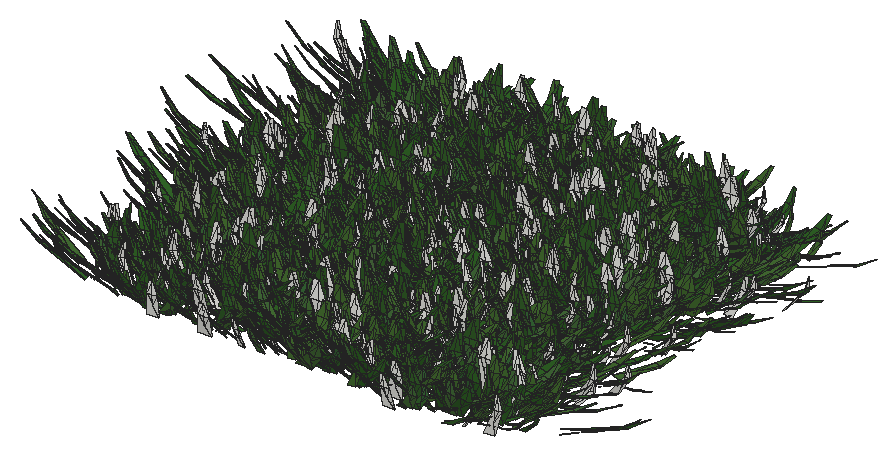
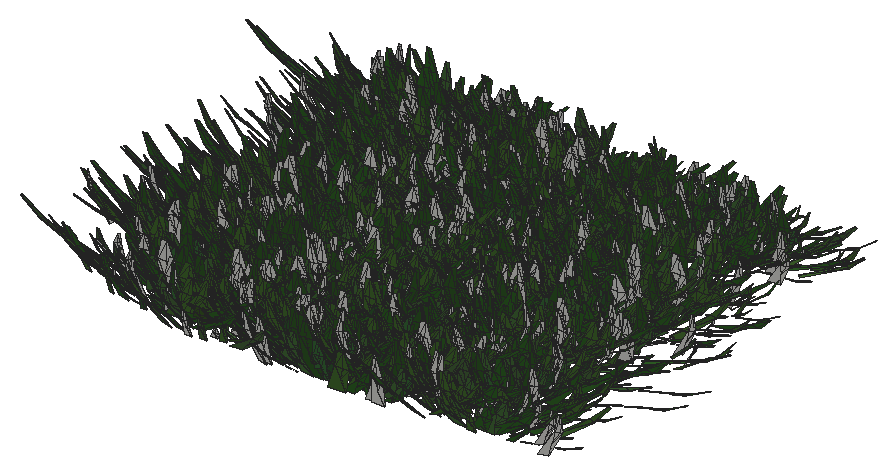
# SketchUp Ruby script. Lengths in inches.
U = 1.inch
M = Sketchup.active_model
def pt(a) = Geom::Point3d.new(a.map { |v| v * U })
def face(e, loops, mat)
  f = e.add_face(loops[0].map { |a| pt(a) })
  loops[1..].each { |l| e.add_face(l.map { |a| pt(a) }).erase! }
  f.material = f.back_material = mat if mat
  f
end
# faces: each face lists its corners as indices into pts; further lists are holes
def faces(e, pts, list, mat = nil) = list.each { |f| face(e, (f[0].is_a?(Array) ? f : [f]).map { |l| l.map { |i| pts[i] } }, mat) }
# xy, xz, yz: faces in a plane at the given z, y or x. An outline is a flat list of corners, or four numbers for a rectangle; further outlines are holes
def ring(l) = l.size == 4 ? [[l[0], l[1]], [l[2], l[1]], [l[2], l[3]], [l[0], l[3]]] : l.each_slice(2).to_a
def flat(e, list, mat, &to3) = list.each { |f| face(e, (f[0].is_a?(Array) ? f : [f]).map { |l| ring(l).map { |u, v| to3.(u, v) } }, mat) }
def xy(e, z, list, mat = nil) = flat(e, list, mat) { |x, y| [x, y, z] }
def xz(e, y, list, mat = nil) = flat(e, list, mat) { |x, z| [x, y, z] }
def yz(e, x, list, mat = nil) = flat(e, list, mat) { |y, z| [x, y, z] }
def lines(e, pts, list) = list.each { |a, b| e.add_line(pt(pts[a]), pt(pts[b])) }
# prism: a flat outline (further loops are holes) pulled along v
def prism(e, loops, v, mat = nil)
  f = face(e, loops, mat); d = Geom::Vector3d.new(v.map { |x| x * U })
  f.pushpull(f.normal.samedirection?(d) ? d.length : -d.length)
end
def box(e, o, s, mat = nil) = prism(e, [[o, [o[0] + s[0], o[1], o[2]], [o[0] + s[0], o[1] + s[1], o[2]], [o[0], o[1] + s[1], o[2]]]], [0, 0, s[2]], mat)
def at(x, y, z, deg = 0) = Geom::Transformation.translation(pt([x, y, z])) * Geom::Transformation.rotation(ORIGIN, Z_AXIS, deg.degrees)
def axes(o, x, y, z) = Geom::Transformation.new([*x, 0, *y, 0, *z, 0, *pt(o).to_a, 1])
def part(name) = M.definitions.add(name)
# library, detail: a bought-in or finely detailed component or shape, given as its bounding box
def library(name, o, s) = part(name).tap { |d| box(d.entities, o, s) }
def detail(e, o, s) = box(e.add_group.entities, o, s)
def put(e, d, t, mat = nil) = e.add_instance(d, t).tap { |i| i.material = mat if mat }
def group(e, t, mat = nil) = e.add_group.tap { |g| g.transformation = t; g.material = mat if mat }.entities
root = M.entities
M.materials.add("Material10").color = [48, 100, 38]
M.materials.add("Material3").color = [68, 110, 58]
M.materials.add("Material4").color = [48, 90, 38]
M.materials.add("Material5").color = [68, 110, 48]
M.materials.add("Material6").color = [48, 90, 48]
M.materials.add("Material7").color = [58, 110, 58]
M.materials.add("Material8").color = [58, 90, 38]
M.materials.add("Material9").color = [68, 100, 58]
c1 = part("grass00")
p = [[-0.6875,0.15,0],[-0.56,0.08,5.52],[-0.04,0.03,2.76],[0.48,-0.02,0],[0.35,-0.02,5.52],[-0.1,-0.14,5.52],
  [-0.12,0.65,8.37],[-0.42,0.65,8.37]]
faces(c1.entities,p,[[0,1,2,3],[3,2,4],[1,5,2],[5,4,2],[1,6,5],[4,5,6],[7,6,1]])
c2 = part("Group16\#1")
put(c2.entities,c1,axes([1.44,-0.61,-0.01],[0.05352,0.12609,0],[-0.10704,0.04543,0.07239],[0.06664,-0.02828,0.11628]),"Material6")
put(c2.entities,c1,axes([0.76,-0.15,-0.01],[0.04676,0.24062,0],[-0.23162,0.04501,0.06642],[0.0652,-0.01267,0.23595]),"Material3")
put(c2.entities,c1,axes([0.79,0.01,-0.01],[-0.00606,0.34651,0],[-0.34381,-0.00602,0.0432],[0.04319,0.00076,0.34386]))
put(c2.entities,c1,axes([1,0.23,-0.01],[-0.07192,0.31144,0],[-0.28722,-0.06632,0.1236],[0.12043,0.02781,0.29478]),"Material5")
put(c2.entities,c1,axes([1.66,0.77,-0.01],[-0.13828,0.29651,0],[-0.21551,-0.1005,0.22471],[0.20365,0.09498,0.23779]),"Material10")
put(c2.entities,c1,axes([0.6875,0.52,-0.01],[-0.18126,0.24051,0],[-0.22746,-0.17142,0.09788],[0.07817,0.05891,0.28481]),"Material5")
put(c2.entities,c1,axes([0.68,0.78,-0.01],[-0.215,0.18688,0],[-0.12385,-0.14248,0.21334],[0.13995,0.16101,0.18878]),"Material3")
put(c2.entities,c1,axes([0.56,1,-0.01],[-0.13756,0.07624,0],[-0.06159,-0.11112,0.0927],[0.04494,0.08108,0.12705]),"Material5")
put(c2.entities,c1,axes([0.2,0.64,-0.01],[-0.23729,0.07254,0],[-0.05711,-0.18681,0.153],[0.04473,0.14632,0.19535]),"Material10")
put(c2.entities,c1,axes([0.0625,0.72,-0.01],[-0.28874,0.02525,0],[-0.02179,-0.24916,0.14647],[0.01276,0.14591,0.25012]),"Material3")
put(c2.entities,c1,axes([-0.08,0.62,-0.01],[-0.34089,-0.04187,0],[0.03255,-0.26504,0.216],[-0.02633,0.21439,0.26703]),"Material10")
put(c2.entities,c1,axes([-0.34,0.98,-0.01],[-0.14314,-0.0493,0],[0.04397,-0.12769,0.06843],[-0.02228,0.0647,0.13505]),"Material10")
put(c2.entities,c1,axes([-0.87,1.45,-0.01],[-0.23488,-0.14114,0],[0.13761,-0.22901,0.06087],[-0.03135,0.05217,0.26717]))
put(c2.entities,c1,axes([-0.72,0.77,-0.01],[-0.14208,-0.13251,0],[0.07209,-0.0773,0.16301],[-0.11118,0.11922,0.1057]),"Material10")
put(c2.entities,c1,axes([-0.62,0.43,-0.01],[-0.14845,-0.21203,0],[0.18654,-0.13061,0.12304],[-0.10079,0.07057,0.22772]),"Material3")
put(c2.entities,c1,axes([-0.68,0.29,-0.01],[-0.13639,-0.32136,0],[0.31723,-0.13464,0.05579],[-0.05136,0.0218,0.34462]),"Material4")
put(c2.entities,c1,axes([-0.64,0.125,-0.01],[-0.0458,-0.23569,0],[0.22124,-0.043,0.08276],[-0.08124,0.01579,0.22538]),"Material7")
put(c2.entities,c1,axes([-1.6,-0.03,-0.01],[0.00576,-0.32897,0],[0.27526,0.00482,0.18018],[-0.18015,-0.00315,0.2753]),"Material5")
put(c2.entities,c1,axes([-1.36,-0.31,-0.01],[0.05718,-0.24765,0],[0.18172,0.04196,0.17267],[-0.16825,-0.03885,0.1865]),"Material10")
put(c2.entities,c1,axes([-1.54,-0.72,-0.01],[0.06537,-0.14017,0],[0.13555,0.06321,0.03939],[-0.0357,-0.01665,0.14956]))
put(c2.entities,c1,axes([-1.19,-0.9,-0.01],[0.09597,-0.12735,0],[0.11214,0.08451,0.07557],[-0.06035,-0.04548,0.14042]),"Material9")
put(c2.entities,c1,axes([-0.47,-0.54,-0.01],[0.11588,-0.10072,0],[0.0618,0.0711,0.12124],[-0.07953,-0.0915,0.0942]))
put(c2.entities,c1,axes([-0.47,-0.84,-0.01],[0.11927,-0.0661,0],[0.06603,0.11913,0.00646],[-0.00313,-0.00565,0.13621]),"Material5")
put(c2.entities,c1,axes([-0.38,-1.24,-0.01],[0.28037,-0.08571,0],[0.0618,0.20215,0.20315],[-0.05939,-0.19428,0.21139]),"Material9")
put(c2.entities,c1,axes([-0.06,-0.66,-0.01],[0.22719,-0.01987,0],[0.01247,0.14255,0.17758],[-0.01547,-0.17691,0.1431]),"Material8")
put(c2.entities,c1,axes([0.11,-0.89,-0.01],[0.14882,0.01828,0],[-0.01058,0.08611,0.12229],[0.01491,-0.12138,0.08676]),"Material6")
put(c2.entities,c1,axes([0.25,-0.72,-0.01],[0.20481,0.07053,0],[-0.06206,0.18022,0.10291],[0.03351,-0.0973,0.1906]),"Material6")
put(c2.entities,c1,axes([0.85,-1.42,-0.01],[0.16481,0.09904,0],[-0.09472,0.15762,0.05616],[0.02893,-0.04814,0.18389]),"Material5")
put(c2.entities,c1,axes([1.01,-1.09,-0.01],[0.21858,0.20385,0],[-0.17495,0.1876,0.15339],[0.10462,-0.11218,0.25652]),"Material10")
put(c2.entities,c1,axes([1.01,-0.71,-0.01],[0.08733,0.12473,0],[-0.06445,0.04512,0.13037],[0.1068,-0.07477,0.07867]),"Material6")
c3 = part("Group15\#1")
put(c3.entities,c2,at(0,0,0))
c4 = part("3darcstudiotree_grass00\#1")
put(c4.entities,c3,at(0,0,0))
put(root,c4,axes([1026.98,934.91,0],[3.5158,-0.29291,0],[1.43894,1.07947,-0.01535],[0.02658,0.01994,1.5577]))
put(root,c4,axes([1028.4,963.98,0],[-3.60429,-0.54918,0],[1.97169,-0.80877,-0.03312],[0.12446,-0.05105,1.70984]))
put(root,c4,axes([1028.05,966.49,0],[1.08767,-1.10089,0],[4.34215,0.26813,-0.04714],[0.21998,0.01358,1.34372]))
put(root,c4,axes([1028.66,944.45,0],[-2.39381,-0.81809,0],[3.41436,-0.62442,-0.02018],[0.11154,-0.0204,1.81061]))
put(root,c4,axes([1027.22,954.21,0],[4.48845,-0.0996,0],[0.40703,1.14637,-0.01913],[0.01094,0.03082,1.86132]))
put(root,c4,axes([1029.08,960.92,0],[-2.33649,-0.74426,0],[3.77896,-0.74146,-0.04646],[0.22132,-0.04342,1.81816]))
put(root,c4,axes([1027.08,970.72,0],[3.85435,0.70628,0],[-2.80826,0.95783,-0.04132],[-0.15487,0.05282,1.88254]))
put(root,c4,axes([1027.89,945.71,0],[-1.94964,1.12405,0],[-4.22902,-0.45845,-0.00354],[-0.01854,-0.00201,1.64409]))
put(root,c4,axes([1027.61,969.89,0],[3.1818,0.67229,0],[-2.74348,0.81152,-0.00305],[-0.01175,0.00348,1.58836]))
put(root,c4,axes([1029.71,961.93,0],[-4.23791,0.69969,0],[-2.41225,-0.91316,-0.01955],[-0.05785,-0.0219,1.46911]))
put(root,c4,axes([1028.93,936.8,0],[3.32161,0.35112,0],[-1.50903,0.89222,-0.04149],[-0.12715,0.07518,1.90578]))
put(root,c4,axes([1028.85,937.58,0],[4.42522,0.39878,0],[-1.59159,1.10387,-0.05978],[-0.10331,0.07165,1.49495]))
put(root,c4,axes([1030.24,933.59,0],[-3.44676,0.28749,0],[-1.23509,-0.92549,-0.01591],[-0.0303,-0.02271,1.46774]))
put(root,c4,axes([1028.71,952.04,0],[3.38445,0.8074,0],[-3.01391,0.7896,-0.00767],[-0.03555,0.00931,1.8325]))
put(root,c4,axes([1029.99,939.57,0],[1.69893,-0.90725,0],[3.27841,0.3837,-0.04141],[0.32735,0.03831,1.97468]))
put(root,c4,axes([1029.22,965.58,0],[3.91819,0.15531,0],[-0.72225,1.13884,-0.02805],[-0.0304,0.04793,1.99488]))
put(root,c4,axes([1030.66,959.5625,0],[-4.474,0.54268,0],[-2.22283,-1.14534,-0.06144],[-0.11475,-0.05913,1.3618]))
put(root,c4,axes([1029.82,948.84,0],[4.53734,-0.32224,0],[1.09679,0.96521,-0.02465],[0.03792,0.03337,1.41248]))
put(root,c4,axes([1031.3,956,0],[-4.98405,0.08955,0],[-0.32681,-1.13684,-0.01837],[-0.00709,-0.02466,1.53349]))
put(root,c4,axes([1030.13,958.07,0],[-2.12527,0.78662,0],[-4.24604,-0.71699,-0.01862],[-0.09082,-0.01534,1.88514]))
put(root,c4,axes([1030.4,947.54,0],[-0.84491,0.92662,0],[-3.59657,-0.20496,-0.03421],[-0.27144,-0.01547,1.87625]))
put(root,c4,axes([1030.09,968.57,0],[4.27273,0.49757,0],[-1.69118,0.90766,-0.0112],[-0.0297,0.01594,1.5714]))
put(root,c4,axes([1030.77,950,0],[-2.09567,1.0755,0],[-4.66144,-0.56769,-0.00711],[-0.02652,-0.00323,1.34501]))
put(root,c4,axes([1031.4375,953.21,0],[3.76579,0.18942,0],[-0.73722,0.91603,-0.0192],[-0.02664,0.0331,1.64321]))
put(root,c4,axes([1033.09,937.56,0],[-4.50451,-0.0411,0],[0.16437,-1.12587,-0.04384],[0.00948,-0.0649,1.66887]))
put(root,c4,axes([1033.57,957.37,0],[1.13978,-1.18562,0],[3.93385,0.23636,-0.00397],[0.02802,0.00168,1.83602]))
put(root,c4,axes([1033.1875,968.22,0],[2.04927,-1.15149,0],[3.67293,0.40854,-0.03607],[0.18559,0.02064,1.41495]))
put(root,c4,axes([1033.99,936.09,0],[-3.89235,0.6193,0],[-1.97046,-0.77403,-0.04609],[-0.18429,-0.07239,1.7083]))
put(root,c4,axes([1034.17,961.06,0],[-4.69047,0.29817,0],[-0.94339,-0.92751,-0.01716],[-0.03313,-0.03258,1.87475]))
put(root,c4,axes([1034.76,939.39,0],[-2.56498,-0.70635,0],[3.60094,-0.81726,-0.05879],[0.23789,-0.05399,1.66118]))
put(root,c4,axes([1033.32,955.72,0],[2.78646,0.69678,0],[-2.91891,0.72956,-0.04694],[-0.21834,0.05457,1.69685]))
put(root,c4,axes([1033.72,951.41,0],[4.00096,-0.34776,0],[1.36846,0.984,-0.02118],[0.04627,0.03327,1.73224]))
put(root,c4,axes([1034.71,934.35,0],[-3.88364,0.22634,0],[-1.16126,-1.24533,-0.06463],[-0.06106,-0.06548,1.33032]))
put(root,c4,axes([1034.99,948.4,0],[-0.3144,-1.12257,0],[4.53452,-0.07937,-0.04142],[0.25114,-0.0044,1.72685]))
put(root,c4,axes([1033.02,959.21,0],[2.22373,1.05105,0],[-4.23729,0.56031,-0.01033],[-0.04653,0.00615,1.52631]))
put(root,c4,axes([1033.55,953.09,0],[1.40015,0.90192,0],[-4.40254,0.42716,-0.04732],[-0.21206,0.02058,1.41896]))
put(root,c4,axes([1035.59,969.95,0],[-2.10821,-0.79686,0],[3.44011,-0.56883,-0.00554],[0.0286,-0.00473,1.59445]))
put(root,c4,axes([1034.11,941.9,0],[-2.15643,1.07136,0],[-4.45067,-0.55989,-0.00338],[-0.01774,-0.00223,1.82725]))
put(root,c4,axes([1035.79,963.875,0],[-1.26196,-1.16235,0],[3.99848,-0.27132,-0.0298],[0.15935,-0.01081,1.43464]))
put(root,c4,axes([1035.8,941.18,0],[-3.90512,0.37554,0],[-1.32571,-0.86161,-0.01112],[-0.02945,-0.01914,1.70172]))
put(root,c4,axes([1034.5,949.9,0],[3.89687,0.53963,0],[-2.2724,1.02562,-0.02111],[-0.06659,0.03005,1.90804]))
put(root,c4,axes([1035.07,946.8125,0],[4.64847,0.14796,0],[-0.47459,0.93187,-0.04636],[-0.04617,0.09067,1.85211]))
put(root,c4,axes([1036.04,965.1875,0],[-3.09239,0.5801,0],[-2.93834,-0.97897,-0.02868],[-0.07819,-0.02605,1.39]))
put(root,c4,axes([1037.25,945.15,0],[-4.25986,-0.54269,0],[2.31668,-1.13655,-0.02171],[0.04865,-0.02387,1.57387]))
put(root,c4,axes([1037.26,954.61,0],[-2.77535,-0.81036,0],[3.4317,-0.73456,-0.03189],[0.13148,-0.02814,1.53238]))
put(root,c4,axes([1036.37,971.45,0],[3.79578,-0.24018,0],[1.14982,1.13575,-0.03471],[0.05624,0.05555,1.93398]))
put(root,c4,axes([1036.91,967.16,0],[-2.12934,0.97427,0],[-4.32415,-0.59067,-0.04785],[-0.24231,-0.0331,1.77706]))
put(root,c4,axes([1036.66,961.58,0],[4.30806,0.2682,0],[-1.01562,1.01959,-0.04825],[-0.06479,0.06504,1.45973]))
put(root,c4,axes([1037.27,944.02,0],[3.59575,0.08404,0],[-0.42601,1.13924,-0.04931],[-0.02468,0.066,1.538]))
put(root,c4,axes([1040.33,945.125,0],[-3.88808,0.63083,0],[-2.21629,-0.85375,-0.02727],[-0.08235,-0.03172,1.41127]))
put(root,c4,axes([1041.2,965.55,0],[-1.09356,-0.98806,0],[3.47695,-0.24051,-0.0133],[0.08295,-0.00574,1.45899]))
put(root,c4,axes([1039.46,961.85,0],[3.11671,0.55561,0],[-2.5205,0.88368,-0.03635],[-0.10975,0.03848,1.41103]))
put(root,c4,axes([1039.84,948.58,0],[1.23042,1.06401,0],[-3.79842,0.27453,-0.04889],[-0.27893,0.02016,1.46761]))
put(root,c4,axes([1041.11,972.26,0],[1.50651,-0.83711,0],[4.29011,0.48255,-0.04402],[0.24827,0.02793,1.81837]))
put(root,c4,axes([1041.9,957.39,0],[-4.37435,-0.52642,0],[1.61836,-0.8405,-0.01121],[0.03956,-0.02054,1.89718]))
put(root,c4,axes([1039.76,960.72,0],[4.06113,0.54294,0],[-1.83498,0.85783,-0.00407],[-0.01255,0.00587,1.59208]))
put(root,c4,axes([1041.53,938.08,0],[1.79956,-0.79311,0],[4.48938,0.63665,-0.03953],[0.18894,0.02679,1.77239]))
put(root,c4,axes([1040.2,936.72,0],[0.4509,1.27151,0],[-4.34293,0.09625,-0.0152],[-0.08927,0.00198,1.60635]))
put(root,c4,axes([1042.55,940.49,0],[0.25819,-1.20405,0],[5.15523,0.06909,-0.00697],[0.04087,0.00055,1.89407]))
put(root,c4,axes([1042.32,943.74,0],[-3.83272,-0.39572,0],[1.58422,-0.959,-0.04671],[0.12739,-0.07712,1.85324]))
put(root,c4,axes([1042.42,971.01,0],[-3.58122,-0.18152,0],[0.97164,-1.19807,-0.02938],[0.02523,-0.03112,1.3208]))
put(root,c4,axes([1041.32,939.16,0],[1.00148,1.21567,0],[-4.0422,0.20812,-0.03105],[-0.22157,0.01141,1.87912]))
put(root,c4,axes([1040.98,966.54,0],[1.9958,1.15638,0],[-4.53864,0.48958,-0.02206],[-0.10786,0.01163,1.64521]))
put(root,c4,axes([1041.61,942.44,0],[1.40221,1.20778,0],[-3.61732,0.26248,-0.03743],[-0.21438,0.01556,1.40382]))
put(root,c4,axes([1042.75,969.3,0],[3.20601,-0.72944,0],[2.8275,0.7767,-0.00947],[0.03301,0.00907,1.36019]))
put(root,c4,axes([1042.15,949.87,0],[2.6445,0.64267,0],[-3.36196,0.86462,-0.04673],[-0.15716,0.04042,1.45453]))
put(root,c4,axes([1042.64,951.25,0],[4.6939,-0.33478,0],[1.42081,1.24507,-0.04256],[0.05609,0.04915,1.55488]))
put(root,c4,axes([1043,952.54,0],[0.70081,1.13515,0],[-3.837,0.14805,-0.04631],[-0.31213,0.01204,1.65491]))
put(root,c4,axes([1042.85,963.16,0],[0.79643,0.97824,0],[-4.073,0.20725,-0.02796],[-0.20539,0.01045,1.94708]))
put(root,c4,axes([1043.52,947.14,0],[4.47521,-0.51509,0],[1.59075,0.86381,-0.00355],[0.00999,0.00542,1.60125]))
put(root,c4,axes([1043.27,955.84,0],[3.61508,0.31151,0],[-1.17398,0.85151,-0.01199],[-0.02287,0.01659,1.31812]))
put(root,c4,axes([1043.49,954.04,0],[1.15853,0.90177,0],[-3.74188,0.30046,-0.04361],[-0.27208,0.02185,1.60948]))
put(root,c4,axes([1043.13,959.61,0],[4.73679,0.47209,0],[-1.3835,0.8676,-0.02018],[-0.04428,0.02777,1.38364]))
put(root,c4,axes([1043.29,968.49,0],[3.02988,0.65339,0],[-2.92725,0.84838,-0.02494],[-0.09513,0.02757,1.63549]))
put(root,c4,axes([1045.28,945.59,0],[-0.26338,-0.96396,0],[4.36475,-0.07454,-0.04502],[0.21373,-0.00365,1.30109]))
put(root,c4,axes([1043.4,934.44,0],[3.70502,0.87773,0],[-2.99978,0.79141,-0.00751],[-0.03439,0.00907,1.8142]))
put(root,c4,axes([1046.42,938.28,0],[1.10203,-1.11719,0],[4.19734,0.25877,-0.00763],[0.05016,0.00309,1.82848]))
put(root,c4,axes([1045.81,971.75,0],[3.66199,-0.54584,0],[2.20621,0.92507,-0.01626],[0.05583,0.02341,1.80561]))
put(root,c4,axes([1047.07,941.99,0],[-2.73315,-0.59238,0],[2.36909,-0.68316,-0.00893],[0.05138,-0.01482,1.98619]))
put(root,c4,axes([1046.53,966.375,0],[2.15048,-1.04444,0],[4.49757,0.57877,-0.06088],[0.28493,0.03667,1.6642]))
put(root,c4,axes([1047.07,961.2,0],[1.29191,-1.13081,0],[3.98569,0.2846,-0.01145],[0.06058,0.00433,1.42532]))
put(root,c4,axes([1047.24,969.75,0],[-3.75042,-0.0193,0],[0.10511,-1.27668,-0.05231],[0.00643,-0.07814,1.90792]))
put(root,c4,axes([1047.02,951.59,0],[2.35649,-0.70912,0],[3.7753,0.78411,-0.00974],[0.03955,0.00821,1.619]))
put(root,c4,axes([1047.42,943.57,0],[-3.90716,-0.09419,0],[0.46436,-1.20386,-0.0118],[0.00503,-0.01303,1.34216]))
put(root,c4,axes([1046.7,946.71,0],[4.63049,-0.46903,0],[1.7734,1.09423,-0.01357],[0.03424,0.02113,1.98263]))
put(root,c4,axes([1046.34,968.41,0],[4.58241,0.19186,0],[-0.7983,1.1917,-0.00046],[-0.00036,0.00053,1.40239]))
put(root,c4,axes([1047.28,954.61,0],[-1.84062,1.15684,0],[-3.44401,-0.34248,-0.04072],[-0.25086,-0.02495,1.53595]))
put(root,c4,axes([1048.23,959.6,0],[-3.43993,-0.35088,0],[1.66399,-1.0196,-0.03312],[0.08822,-0.05406,1.94116]))
put(root,c4,axes([1046.69,934.34,0],[3.69288,0.11707,0],[-0.52356,1.03223,-0.01144],[-0.00941,0.01856,1.7012]))
put(root,c4,axes([1047.26,965.53,0],[4.06672,-0.35788,0],[1.7117,1.21566,-0.03514],[0.05649,0.04012,1.55988]))
put(root,c4,axes([1047.01,939.72,0],[3.74539,0.69391,0],[-2.4561,0.82855,-0.03152],[-0.10739,0.03623,1.47514]))
put(root,c4,axes([1049.3,936.01,0],[-1.01831,-1.20571,0],[4.14332,-0.21871,-0.00703],[0.03921,-0.00207,1.50812]))
put(root,c4,axes([1047.77,947.94,0],[4.09573,-0.25172,0],[0.94943,0.96549,-0.02888],[0.04811,0.04892,1.73467]))
put(root,c4,axes([1049.53,941.26,0],[-2.36855,-0.74824,0],[3.41575,-0.67578,-0.00813],[0.03094,-0.00612,1.32168]))
put(root,c4,axes([1048.1,957.9,0],[-0.73359,1.07978,0],[-4.59667,-0.19518,-0.06003],[-0.37487,-0.01592,1.84592]))
put(root,c4,axes([1049.63,963.13,0],[-2.50204,-0.67667,0],[3.03986,-0.70251,-0.01026],[0.05042,-0.01165,1.73127]))
put(root,c4,axes([1047.78,952.99,0],[2.78719,0.78007,0],[-2.78295,0.62147,-0.01423],[-0.0832,0.01858,1.82816]))
put(root,c4,axes([1049.53,961.86,0],[1.6891,-0.96656,0],[4.41238,0.48192,-0.02716],[0.12133,0.01325,1.46706]))
put(root,c4,axes([1048,955.8,0],[1.88303,0.87084,0],[-3.91676,0.52933,-0.00296],[-0.01453,0.00196,1.55057]))
put(root,c4,axes([1048.89,950.55,0],[-2.57647,0.98803,0],[-3.47817,-0.56688,-0.00573],[-0.03032,-0.00494,1.63969]))
put(root,c4,axes([1051.18,950.33,0],[-3.28034,-0.7048,0],[2.67551,-0.77829,-0.00129],[0.00481,-0.0014,1.46122]))
put(root,c4,axes([1051.58,935.26,0],[-4.50482,0.23028,0],[-0.80598,-0.98543,-0.0347],[-0.04459,-0.05452,1.61275]))
put(root,c4,axes([1052.05,972.34,0],[-2.24979,-0.88649,0],[3.27379,-0.51928,-0.00968],[0.0585,-0.00928,1.73508]))
put(root,c4,axes([1051.84,955.12,0],[-2.16564,-0.83911,0],[3.14801,-0.50779,-0.04434],[0.21001,-0.03388,1.31982]))
put(root,c4,axes([1052.22,969.36,0],[-0.67756,-0.92885,0],[4.95794,-0.22604,-0.01194],[0.05933,-0.0027,1.59034]))
put(root,c4,axes([1052.95,945.39,0],[-1.3799,-0.92069,0],[4.85694,-0.45496,-0.00645],[0.02452,-0.0023,1.31612]))
put(root,c4,axes([1052.17,962.58,0],[-3.11177,0.67846,0],[-2.86968,-0.82262,-0.0546],[-0.24326,-0.06973,1.84968]))
put(root,c4,axes([1051.21,939.92,0],[0.29202,1.19913,0],[-4.14046,0.06302,-0.02381],[-0.16303,0.00248,1.77807]))
put(root,c4,axes([1052.57,946.625,0],[0.24548,-1.00327,0],[4.53075,0.06929,-0.05271],[0.25543,0.00391,1.37729]))
put(root,c4,axes([1052.32,935.82,0],[2.19726,-0.80915,0],[3.02534,0.51346,-0.03969],[0.20361,0.03456,1.41714]))
put(root,c4,axes([1052.35,963.13,0],[-3.397,0.74366,0],[-2.61152,-0.74558,-0.00238],[-0.01206,-0.00344,1.90825]))
put(root,c4,axes([1053.31,944.39,0],[-3.12263,-0.80969,0],[2.7475,-0.66225,-0.03577],[0.16124,-0.03886,1.49339]))
put(root,c4,axes([1051.96,942.45,0],[1.11929,0.91122,0],[-4.49159,0.34483,-0.03259],[-0.18787,0.01442,1.77089]))
put(root,c4,axes([1052.06,967.72,0],[0.31588,1.13425,0],[-4.04106,0.07034,-0.01352],[-0.07984,0.00139,1.49862]))
put(root,c4,axes([1051.96,952.07,0],[3.21264,0.8518,0],[-2.81244,0.66296,-0.02839],[-0.16121,0.038,1.88589]))
put(root,c4,axes([1054.06,949,0],[-0.18941,-0.91577,0],[4.95051,-0.06399,-0.00424],[0.02167,-0.00028,1.58408]))
put(root,c4,axes([1054.36,970.76,0],[-4.97788,-0.34272,0],[1.27823,-1.16037,-0.00177],[0.00271,-0.00246,1.73275]))
put(root,c4,axes([1053.12,960.84,0],[3.21803,-0.64979,0],[2.61533,0.80951,-0.03491],[0.156,0.04829,1.84986]))
put(root,c4,axes([1053.31,965.49,0],[-2.15492,0.7494,0],[-3.61151,-0.64906,-0.0015],[-0.00592,-0.00106,1.35234]))
put(root,c4,axes([1055.3,940.9,0],[-4.78225,-0.48138,0],[1.79554,-1.11486,-0.01703],[0.03477,-0.02159,1.64249]))
put(root,c4,axes([1054.74,933.73,0],[-3.37934,0.52143,0],[-1.92704,-0.78055,-0.03387],[-0.1051,-0.04257,1.3548]))
put(root,c4,axes([1055.31,952.92,0],[-4.43307,0.16391,0],[-0.66186,-1.11881,-0.04443],[-0.04202,-0.07104,1.82802]))
put(root,c4,axes([1053.71,937.8,0],[3.59313,0.68873,0],[-2.26385,0.73816,-0.03117],[-0.10632,0.03467,1.30357]))
put(root,c4,axes([1053.91,966.77,0],[-0.883,1.08324,0],[-4.56364,-0.2325,-0.00834],[-0.04858,-0.00247,1.72954]))
put(root,c4,axes([1055.21,956.46,0],[3.26656,-0.94634,0],[3.22899,0.69661,-0.04774],[0.259,0.05588,1.91023]))
put(root,c4,axes([1054.375,957.27,0],[1.182,1.03878,0],[-4.83466,0.34383,-0.01266],[-0.06647,0.00473,1.71446]))
put(root,c4,axes([1055.25,959.23,0],[3.68181,-0.04873,0],[0.19766,0.93331,-0.02933],[0.01311,0.06192,1.97542]))
put(root,c4,axes([1057.52,948.97,0],[-3.47365,-0.63097,0],[2.73432,-0.94081,-0.03763],[0.14803,-0.05093,1.94544]))
put(root,c4,axes([1057.88,942.57,0],[-3.67495,-0.82991,0],[3.18036,-0.88019,-0.0585],[0.25242,-0.06986,1.90866]))
put(root,c4,axes([1057.73,954.53,0],[1.84359,-0.98578,0],[4.27522,0.49972,-0.01397],[0.07469,0.00873,1.74087]))
put(root,c4,axes([1058.36,960.96,0],[-2.66867,-0.63345,0],[3.02701,-0.79703,-0.01822],[0.08532,-0.02247,1.86907]))
put(root,c4,axes([1057.24,947.52,0],[-1.38022,0.90937,0],[-3.69449,-0.35046,-0.03389],[-0.21225,-0.02013,1.65454]))
put(root,c4,axes([1058.54,935.1875,0],[-3.71907,-0.26708,0],[1.32824,-1.15597,-0.05258],[0.08896,-0.07742,1.84274]))
put(root,c4,axes([1059.07,961.74,0],[-3.44494,-0.92514,0],[2.808,-0.65351,-0.04944],[0.24269,-0.05648,1.60821]))
put(root,c4,axes([1058.09,971.24,0],[-1.24544,1.08485,0],[-3.56774,-0.25599,-0.04255],[-0.31037,-0.02227,1.76068]))
put(root,c4,axes([1059.01,940.36,0],[-0.08294,-1.02259,0],[4.8002,-0.02433,-0.05384],[0.23738,-0.0012,1.32332]))
put(root,c4,axes([1058.98,943.83,0],[-3.9311,-0.05315,0],[0.20584,-0.95146,-0.00522],[0.00166,-0.00767,1.40302]))
put(root,c4,axes([1059.0625,951.93,0],[-4.14008,0.40448,0],[-1.31245,-0.8396,-0.02866],[-0.08715,-0.05575,1.88291]))
put(root,c4,axes([1059.9,945.9,0],[-3.68165,-0.61094,0],[2.8571,-1.07609,-0.03911],[0.09635,-0.03629,1.43856]))
put(root,c4,axes([1059.29,939.05,0],[-0.00357,-0.95329,0],[3.72251,-0.00087,-0.0371],[0.29437,-0.00007,1.84609]))
put(root,c4,axes([1060.15,952.89,0],[-3.07811,-0.52655,0],[2.38746,-0.87229,-0.01797],[0.0526,-0.01922,1.36964]))
put(root,c4,axes([1059.14,938.36,0],[3.95966,-0.70893,0],[2.92387,1.02069,-0.04389],[0.15667,0.05469,1.92393]))
put(root,c4,axes([1060.78,963.54,0],[-2.20402,-1.1259,0],[4.50927,-0.5517,-0.06506],[0.31838,-0.03895,1.70958]))
put(root,c4,axes([1060.65,958.6,0],[1.30701,-0.93257,0],[4.74609,0.41573,-0.02001],[0.10664,0.00934,1.77455]))
put(root,c4,axes([1060.31,964.94,0],[2.24839,-0.79603,0],[3.33272,0.58833,-0.00946],[0.04896,0.00864,1.61646]))
put(root,c4,axes([1059.49,969.53,0],[-1.06084,1.03088,0],[-4.97495,-0.31997,-0.03008],[-0.16035,-0.01031,1.76703]))
put(root,c4,axes([1059.25,956.27,0],[3.29499,0.88006,0],[-3.34052,0.78169,-0.05678],[-0.19382,0.04535,1.337]))
put(root,c4,axes([1060.29,936.79,0],[4.12637,-0.29278,0],[1.25845,1.1085,-0.03157],[0.05307,0.04674,1.77323]))
